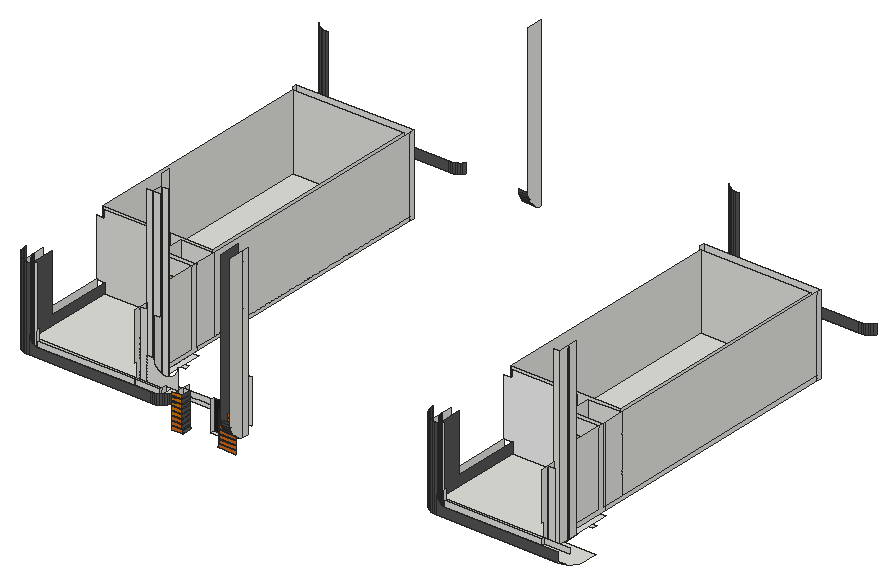
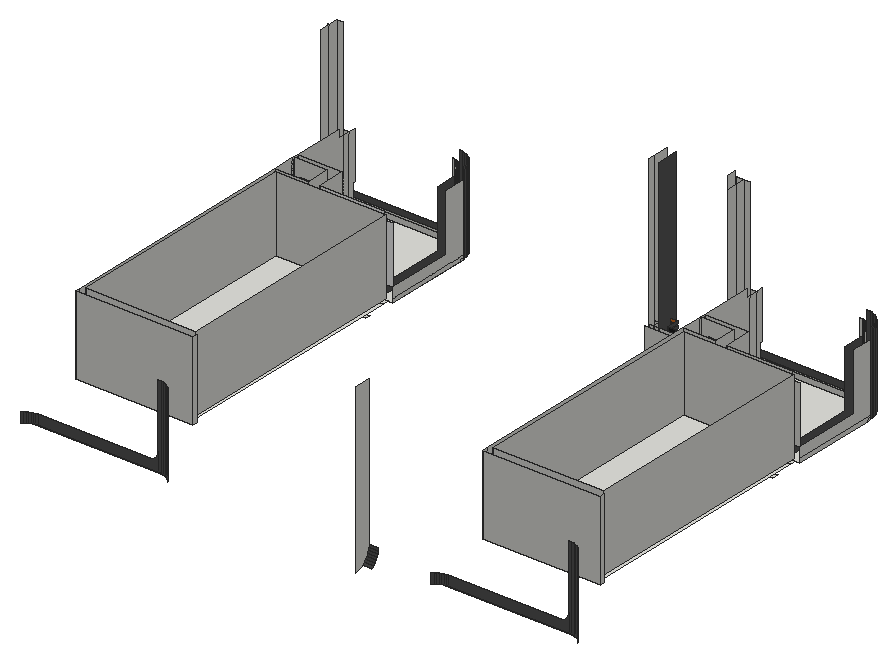
# SketchUp Ruby script. Lengths in inches.
U = 1.inch
M = Sketchup.active_model
def pt(a) = Geom::Point3d.new(a.map { |v| v * U })
def face(e, loops, mat)
  f = e.add_face(loops[0].map { |a| pt(a) })
  loops[1..].each { |l| e.add_face(l.map { |a| pt(a) }).erase! }
  f.material = f.back_material = mat if mat
  f
end
# faces: each face lists its corners as indices into pts; further lists are holes
def faces(e, pts, list, mat = nil) = list.each { |f| face(e, (f[0].is_a?(Array) ? f : [f]).map { |l| l.map { |i| pts[i] } }, mat) }
# xy, xz, yz: faces in a plane at the given z, y or x. An outline is a flat list of corners, or four numbers for a rectangle; further outlines are holes
def ring(l) = l.size == 4 ? [[l[0], l[1]], [l[2], l[1]], [l[2], l[3]], [l[0], l[3]]] : l.each_slice(2).to_a
def flat(e, list, mat, &to3) = list.each { |f| face(e, (f[0].is_a?(Array) ? f : [f]).map { |l| ring(l).map { |u, v| to3.(u, v) } }, mat) }
def xy(e, z, list, mat = nil) = flat(e, list, mat) { |x, y| [x, y, z] }
def xz(e, y, list, mat = nil) = flat(e, list, mat) { |x, z| [x, y, z] }
def yz(e, x, list, mat = nil) = flat(e, list, mat) { |y, z| [x, y, z] }
def lines(e, pts, list) = list.each { |a, b| e.add_line(pt(pts[a]), pt(pts[b])) }
# prism: a flat outline (further loops are holes) pulled along v
def prism(e, loops, v, mat = nil)
  f = face(e, loops, mat); d = Geom::Vector3d.new(v.map { |x| x * U })
  f.pushpull(f.normal.samedirection?(d) ? d.length : -d.length)
end
def box(e, o, s, mat = nil) = prism(e, [[o, [o[0] + s[0], o[1], o[2]], [o[0] + s[0], o[1] + s[1], o[2]], [o[0], o[1] + s[1], o[2]]]], [0, 0, s[2]], mat)
def at(x, y, z, deg = 0) = Geom::Transformation.translation(pt([x, y, z])) * Geom::Transformation.rotation(ORIGIN, Z_AXIS, deg.degrees)
def axes(o, x, y, z) = Geom::Transformation.new([*x, 0, *y, 0, *z, 0, *pt(o).to_a, 1])
def part(name) = M.definitions.add(name)
# library, detail: a bought-in or finely detailed component or shape, given as its bounding box
def library(name, o, s) = part(name).tap { |d| box(d.entities, o, s) }
def detail(e, o, s) = box(e.add_group.entities, o, s)
def put(e, d, t, mat = nil) = e.add_instance(d, t).tap { |i| i.material = mat if mat }
def group(e, t, mat = nil) = e.add_group.tap { |g| g.transformation = t; g.material = mat if mat }.entities
root = M.entities
M.materials.add("[0039_DarkOrange]").color = [219, 120, 0]
M.materials.add("[0041_Chocolate]").color = [210, 105, 30]
M.materials.add("[0129_WhiteSmoke]").color = [245, 245, 245]
M.materials.add("[Color M06]").color = [84, 84, 84]
M.materials.add("[Color M08]").color = [30, 30, 30]
c1 = library("元件\#5",[-4.39,0,0],[5.37,35.83,90.55])
xy(root,90.875,[[897.21,280.47,915.39,281.47],[969.37,280.47,998.64,281.47]],"[0041_Chocolate]")
xy(root,95.51,[[684.87,439.98,732.5,448.51],[1335.37,439.98,1383,448.51]])
xy(root,95.83,[[897.21,280.47,913.53,281.47],[971.24,280.47,998.64,281.47]],"[0041_Chocolate]")
xy(root,97.27,[[946.98,295.65,971.43,300.34]])
xy(root,97.9375,[[897.21,280.47,913.25,281.47],[971.52,280.47,998.64,281.47]],"[0041_Chocolate]")
xy(root,101.1875,[[777.42,397.86,824.61,405.05],[1427.92,397.86,1475.11,405.05]])
xy(root,102.89,[[897.21,280.47,912.6,281.47],[972.17,280.47,998.64,281.47]],"[0041_Chocolate]")
xy(root,105,[[897.21,280.47,912.6,281.47],[972.17,280.47,998.64,281.47]],"[0041_Chocolate]")
xy(root,109.9375,[[984.18,299.11,999.52,302.46]])
xy(root,109.95,[[897.21,280.47,912.6,281.47],[972.17,280.47,998.64,281.47]],"[0041_Chocolate]")
xy(root,112.0625,[[897.21,280.47,912.6,281.47]],"[0039_DarkOrange]")
xy(root,112.0625,[[972.17,280.47,998.64,281.47]],"[0041_Chocolate]")
xy(root,117.02,[[897.21,280.47,912.6,281.47]],"[0039_DarkOrange]")
xy(root,117.02,[[972.17,280.47,998.64,281.47]],"[0041_Chocolate]")
xy(root,119.125,[[897.21,280.47,912.6,281.47]],"[0039_DarkOrange]")
xy(root,119.125,[[972.17,280.47,998.64,281.47]],"[0041_Chocolate]")
xy(root,124.08,[[897.21,280.47,912.6,281.47]],"[0039_DarkOrange]")
xy(root,124.08,[[972.17,280.47,998.64,281.47]],"[0041_Chocolate]")
xy(root,126.125,[[679.54,267.75,675.54,268.01,671.61,268.79,669.16,269.625,881.95,269.625,878.9,268.59,875.73,267.96,872.51,267.75],[1330.04,267.75,1326.04,268.01,1322.11,268.79,1319.66,269.625,1532.45,269.625,1529.4,268.59,1526.23,267.96,1523.01,267.75],[669.16,269.625,667.8125,270.08,664.22,271.85,660.88,274.08,657.87,276.72,656.13,278.71,655.23,279.74,653,283.07,651.23,286.66,649.94,290.46,649.16,294.39,648.9,298.39,648.9,439.98,767.38,439.98,767.38,397.86,836,397.86,836,305.58,845.71,305.58,845.71,312.8125,897.21,312.8125,897.21,305.58,896.71,305.58,896.71,292.45,897.21,292.45,897,289.23,896.37,286.06,895.33,283,893.9,280.1,892.11,277.41,889.98,274.98,887.55,272.85,884.86,271.06,881.96,269.63,881.95,269.625],[1319.66,269.625,1318.3125,270.08,1314.72,271.85,1311.38,274.08,1308.37,276.72,1306.63,278.71,1305.73,279.74,1303.5,283.07,1301.73,286.66,1300.44,290.46,1299.66,294.39,1299.4,298.39,1299.4,439.98,1417.88,439.98,1417.88,397.86,1486.5,397.86,1486.5,305.58,1496.21,305.58,1496.21,312.8125,1547.71,312.8125,1547.71,305.58,1547.21,305.58,1547.21,292.45,1547.71,292.45,1547.5,289.23,1546.87,286.06,1545.83,283,1544.4,280.1,1542.61,277.41,1540.48,274.98,1538.05,272.85,1535.36,271.06,1532.46,269.63,1532.45,269.625],[896.71,292.45,897.21,302.46],
  [896.71,302.46,897.21,305.58],[836,305.58,845.71,312.8125],[1486.5,305.58,1496.21,312.8125],[836,312.8125,845.71,397.86],[845.71,312.8125,846.02,321.34],
  [846.02,312.8125,847.59,321.34],[847.59,312.8125,857.24,321.34],[857.24,312.8125,897.21,321.34],[1486.5,312.8125,1496.21,397.86],[1496.21,312.8125,1496.52,321.34],
  [1496.52,312.8125,1498.09,321.34],[845.71,321.34,846.02,336.27],[846.02,321.34,847.59,336.27],[1496.21,321.34,1496.52,336.27],[1496.52,321.34,1498.09,336.27],
  [767.38,397.86,786.21,397.86,786.21,448.51,656.13,448.51,656.13,439.98,767.38,439.98],[786.21,397.86,836,406.38],[1417.88,397.86,1436.71,397.86,1436.71,448.51,1306.63,448.51,1306.63,439.98,1417.88,439.98],[1436.71,397.86,1486.5,406.38],[786.21,406.38,836,830.91],
  [1436.71,406.38,1486.5,830.91],[656.13,448.51,786.21,830.91],[1306.63,448.51,1436.71,830.91],[648.9,830.91,836,838.14],[1299.4,830.91,1486.5,838.14],
  [602.85,958.64,598.85,958.91,594.92,959.6875,592.47,960.52,805.26,960.52,802.22,959.49,799.05,958.86,795.82,958.64],[1258.35,958.64,1254.35,958.91,1250.42,959.6875,1247.97,960.52,1460.76,960.52,1457.72,959.49,1454.55,958.86,1451.32,958.64]])
xy(root,126.1875,[[897.21,280.47,912.6,281.47]],"[0039_DarkOrange]")
xy(root,126.1875,[[972.17,280.47,998.64,281.47]],"[0041_Chocolate]")
xy(root,128.75,[[648.9,294.33,661.9,305.58],[1299.4,294.33,1312.4,305.58]])
xy(root,131.14,[[897.21,280.47,912.6,281.47]],"[0039_DarkOrange]")
xy(root,131.14,[[972.17,280.47,998.64,281.47]],"[0041_Chocolate]")
xy(root,132.47,[[679.54,281.47,679.54,285.84,836,285.84,836,395.98,824.61,395.98,824.61,403.17,777.42,403.17,777.42,395.98,765.68,395.98,765.68,439.98,662.61,439.98,662.61,298.39,662.76,296.18,663.1875,294.01,663.9,291.91,664.88,289.93,666.11,288.09,667.57,286.42,669.23,284.96,671.07,283.73,673.06,282.75,675.16,282.04,677.33,281.61],[679.54,281.47,836,285.84],[836,281.47,876.59,285.84],[1330.04,281.47,1330.04,285.84,1486.5,285.84,1486.5,395.98,1475.11,395.98,1475.11,403.17,1427.92,403.17,1427.92,395.98,1416.18,395.98,1416.18,439.98,1313.11,439.98,1313.11,298.39,1313.26,296.18,1313.6875,294.01,1314.4,291.91,1315.38,289.93,1316.61,288.09,1318.07,286.42,1319.73,284.96,1321.57,283.73,1323.56,282.75,1325.66,282.04,1327.83,281.61],[1330.04,281.47,1486.5,285.84],
  [836,285.84,876.59,292.45],[836,292.45,876.59,312.8125],[783.26,403.17,836,439.98],[1433.76,403.17,1486.5,439.98],[654.4,445.49,830.5,825.41],
  [1304.9,445.49,1481,825.41]])
xy(root,133.25,[[897.21,280.47,912.6,281.47]],"[0039_DarkOrange]")
xy(root,133.25,[[972.17,280.47,998.64,281.47]],"[0041_Chocolate]")
xy(root,138.2,[[897.21,280.47,912.6,281.47]],"[0039_DarkOrange]")
xy(root,138.2,[[972.17,280.47,998.64,281.47]],"[0041_Chocolate]")
xy(root,140.3125,[[897.21,280.47,912.6,281.47]],"[0039_DarkOrange]")
xy(root,140.3125,[[972.17,280.47,998.64,281.47]],"[0041_Chocolate]")
xz(root,267.75,[[679.54,126.125,872.51,126.125,872.51,141.26,692.98,141.26,691.2,141.46,689.46,141.89,687.79,142.53,686.21,143.38,684.75,144.42,683.43,145.64,682.28,147.01,681.32,148.52,680.55,150.14,679.99,151.84,679.65,153.6,679.54,155.39],[1330.04,126.125,1523.01,126.125,1523.01,141.26,1343.48,141.26,1341.7,141.46,1339.96,141.89,1338.29,142.53,1336.71,143.38,1335.25,144.42,1333.93,145.64,1332.78,147.01,1331.82,148.52,1331.05,150.14,1330.49,151.84,1330.15,153.6,1330.04,155.39]],"[Color M06]")
xz(root,280.47,[[897.21,112.0625,912.6,117.02],[897.21,119.125,912.6,124.08],[897.21,126.1875,912.6,131.14],[897.21,133.25,912.6,138.2],[897.21,140.3125,912.6,145.27]],"[0039_DarkOrange]")
xz(root,280.47,[[897.21,90.875,915.39,90.875,913.61,95.18,913.53,95.83,897.21,95.83],[969.37,90.875,998.64,90.875,998.64,95.83,971.24,95.83,971.16,95.18],[897.21,97.9375,913.25,97.9375,912.6,102.89,897.21,102.89],[971.52,97.9375,998.64,97.9375,998.64,102.89,972.17,102.89],[897.21,105,912.6,109.95],
  [972.17,105,998.64,109.95],[972.17,112.0625,998.64,117.02],[972.17,119.125,998.64,124.08],[972.17,126.1875,998.64,131.14],[972.17,133.25,998.64,138.2],
  [972.17,140.3125,998.64,145.27]],"[0041_Chocolate]")
xz(root,281.47,[[679.54,132.47,836,141.26],[836,132.47,876.59,141.26],[1330.04,132.47,1486.5,141.26]])
xz(root,281.47,[[897.21,117.02,912.6,119.125],[897.21,124.08,912.6,126.1875],[897.21,131.14,912.6,133.25],[897.21,138.2,912.6,140.3125]],"[0039_DarkOrange]")
xz(root,281.47,[[897.21,95.83,913.53,95.83,913.25,97.9375,897.21,97.9375],[971.24,95.83,998.64,95.83,998.64,97.9375,971.52,97.9375],[897.21,102.89,912.6,105],[972.17,102.89,998.64,105],[897.21,109.95,912.6,112.0625],
  [972.17,109.95,998.64,112.0625],[972.17,117.02,998.64,119.125],[972.17,124.08,998.64,126.1875],[972.17,131.14,998.64,133.25],[972.17,138.2,998.64,140.3125]],"[0041_Chocolate]")
xz(root,285.84,[[679.54,132.47,876.59,141.26],[1330.04,132.47,1527.09,141.26]])
xz(root,292.45,[[991.85,126.125,992.73,141.26],[992.73,126.125,998.64,141.26],[836,132.47,847.59,240.16],[847.59,132.47,876.59,132.47,876.59,141.26,897.21,141.26,897.21,174.51,897.18,173.46,897.1,172.42,896.96,171.38,896.77,170.36,896.53,169.34,896.23,168.33,895.88,167.35,895.48,166.38,895.03,165.4375,894.53,164.52,893.99,163.625,893.39,162.76,892.76,161.93,892.08,161.14,891.36,160.38,890.6,159.66,889.8,158.98,888.97,158.34,888.11,157.75,887.22,157.2,886.3,156.7,885.36,156.25,884.39,155.85,883.4,155.5,882.4,155.21,881.38,154.96,880.35,154.77,879.32,154.64,878.27,154.55,877.23,154.53,876.18,154.55,875.14,154.64,874.1,154.77,873.07,154.96,872.05,155.21,871.05,155.5,870.07,155.85,869.1,156.25,868.15,156.7,867.23,157.2,866.34,157.75,865.48,158.34,864.65,158.98,863.85,159.66,863.1,160.38,862.375,161.14,861.7,161.93,861.06,162.76,860.47,163.625,859.92,164.52,859.42,165.4375,858.97,166.38,858.57,167.35,858.22,168.33,857.92,169.34,857.68,170.36,857.49,171.38,857.35,172.42,857.27,173.46,857.24,174.51,847.59,174.51],[1486.5,132.47,1498.09,240.16]])
xz(root,295.65,[[971.43,97.27,972.17,97.27,972.17,102.89,971.52,97.9375]])
xz(root,300.34,[[946.98,97.27,971.43,97.27,971.52,97.9375,972.17,102.89,972.17,145.27,946.98,145.27]],"[Color M08]")
xz(root,302.46,[[896.71,95.62,897.21,126.125],[984.18,109.9375,991.85,126.125],[991.85,109.9375,992.73,126.125],[992.73,109.9375,999.52,126.125],[897.21,126.125,984.18,132.47],
  [984.18,126.125,991.85,132.47],[991.85,126.125,992.73,132.47],[992.73,126.125,999.52,132.47],[897.21,132.47,984.18,141.26],[984.18,132.47,991.85,141.26],
  [991.85,132.47,992.73,141.26],[992.73,132.47,999.52,141.26]])
xz(root,305.58,[[836,126.125,845.71,402.64],[845.71,126.125,847.59,126.125,847.59,226.8,857.24,226.8,857.24,402.64,845.71,402.64],[1486.5,126.125,1496.21,402.64]])
xz(root,312.8125,[[836,126.125,897.21,132.47]])
xz(root,321.34,[[845.71,126.125,847.59,402.64],[847.59,126.125,857.24,402.64],[1496.21,126.125,1498.09,402.64]])
xz(root,343.15,[[937.76,96.14,974.45,165.14]])
xz(root,395.98,[[765.68,132.47,777.42,132.47,777.42,227.53,824.61,227.53,824.61,132.47,836,132.47,836,252.47,765.68,252.47],[1416.18,132.47,1427.92,132.47,1427.92,227.53,1475.11,227.53,1475.11,132.47,1486.5,132.47,1486.5,252.47,1416.18,252.47]])
xz(root,403.17,[[777.42,132.47,783.26,227.53],[783.26,132.47,824.61,227.53],[824.61,132.47,824.61,227.53,783.26,227.53,783.26,252.47,836,252.47,836,132.47],[1427.92,132.47,1433.76,227.53],[1433.76,132.47,1475.11,227.53],
  [1475.11,132.47,1475.11,227.53,1433.76,227.53,1433.76,252.47,1486.5,252.47,1486.5,132.47]])
xz(root,439.98,[[662.61,132.47,765.68,132.47,765.68,252.47,662.61,252.47,662.61,240.16,648.9,240.16,648.9,148.66,662.61,148.66],[783.26,132.47,836,252.47],[1433.76,132.47,1486.5,252.47]])
xz(root,439.98,[[1313.11,132.47,1416.18,132.47,1416.18,252.47,1313.11,252.47,1313.11,240.16,1299.4,240.16,1299.4,148.66,1313.11,148.66]],"[0129_WhiteSmoke]")
xz(root,445.49,[[654.4,132.47,830.5,252.47],[1304.9,132.47,1481,252.47]])
xz(root,825.41,[[654.4,132.47,830.5,252.47],[1304.9,132.47,1481,252.47]])
xz(root,838.14,[[648.9,126.125,836,252.47],[1299.4,126.125,1486.5,252.47]])
xz(root,958.64,[[602.85,126.125,795.82,126.125,795.82,141.26,616.29,141.26,614.51,141.46,612.77,141.89,611.1,142.53,609.52,143.38,608.0625,144.42,606.75,145.64,605.6,147.01,604.63,148.52,603.86,150.14,603.3,151.84,602.96,153.6,602.85,155.39],[1258.35,126.125,1451.32,126.125,1451.32,141.26,1271.79,141.26,1270.01,141.46,1268.27,141.89,1266.6,142.53,1265.02,143.38,1263.5625,144.42,1262.25,145.64,1261.1,147.01,1260.13,148.52,1259.36,150.14,1258.8,151.84,1258.46,153.6,1258.35,155.39]],"[Color M06]")
yz(root,648.9,[[298.39,126.125,305.58,128.75],[305.58,126.125,305.58,128.75,298.39,128.75,298.39,132.47,439.98,132.47,439.98,126.125],[830.91,126.125,838.14,252.47],[298.39,132.47,298.39,240.16,333.33,240.16,333.33,148.66,439.98,148.66,439.98,132.47]])
yz(root,654.4,[[445.49,132.47,825.41,252.47]])
yz(root,662.61,[[298.39,132.47,439.98,132.47,439.98,148.66,333.33,148.66,333.33,240.16,298.39,240.16]],"[Color M06]")
yz(root,679.54,[[281.47,132.47,285.84,155.39]])
yz(root,765.68,[[395.98,132.47,439.98,252.47]])
yz(root,777.42,[[395.98,132.47,403.17,227.53]])
yz(root,783.26,[[403.17,132.47,439.98,252.47]])
yz(root,824.61,[[395.98,132.47,403.17,227.53]])
yz(root,830.5,[[445.49,132.47,825.41,252.47]])
yz(root,836,[[312.8125,126.125,312.8125,132.47,395.98,132.47,395.98,252.47,403.17,252.47,403.17,132.47,406.38,132.47,406.38,126.125],[406.38,126.125,830.91,132.47],[830.91,126.125,838.14,252.47],[281.47,132.47,281.47,141.26,285.84,141.26,285.84,163.7,281.47,163.7,281.47,240.16,292.45,240.16,292.45,132.47],[292.45,132.47,305.58,240.16],
  [305.58,132.47,305.58,240.16,312.8125,240.16,312.8125,252.47,395.98,252.47,395.98,132.47],[403.17,132.47,406.38,252.47],[406.38,132.47,439.98,252.47],[439.98,132.47,830.91,252.47]])
yz(root,845.71,[[305.58,126.125,321.34,402.64],[321.34,126.125,337.5625,402.64]])
yz(root,847.59,[[321.34,126.125,336.27,421.25]])
yz(root,876.59,[[281.47,132.47,285.84,141.26],[285.84,132.47,292.45,141.26]])
yz(root,896.71,[[302.46,95.62,305.58,126.125]])
yz(root,897.21,[[292.45,126.125,302.46,141.26],[302.46,126.125,305.58,132.47],[305.58,126.125,312.8125,132.47],[302.46,132.47,305.58,141.26],[305.58,132.47,312.8125,141.26]])
yz(root,912.6,[[281.47,102.89,295.65,105],[280.47,105,295.65,109.95],[281.47,109.95,295.65,112.0625],[280.47,112.0625,295.65,117.02],[281.47,117.02,295.65,119.125],
  [280.47,119.125,295.65,124.08],[281.47,124.08,295.65,126.1875],[280.47,126.1875,295.65,131.14],[281.47,131.14,295.65,133.25],[280.47,133.25,295.65,138.2],
  [281.47,138.2,295.65,140.3125],[280.47,140.3125,295.65,145.27]],"[Color M06]")
yz(root,922.83,[[983.34,110.72,983.34,376.875,958.64,376.875,958.64,141.3,958.91,137.2,959.71,133.18,961.03,129.3,962.85,125.62,965.125,122.21,967.83,119.12,970.91,116.42,974.32,114.14,978,112.32,981.89,111.01]])
yz(root,946.98,[[295.65,97.27,300.34,145.27]])
yz(root,972.17,[[281.47,102.89,300.34,105],[280.47,105,300.34,109.95],[281.47,109.95,300.34,112.0625],[280.47,112.0625,300.34,117.02],[281.47,117.02,300.34,119.125],
  [280.47,119.125,300.34,124.08],[281.47,124.08,300.34,126.1875],[280.47,126.1875,300.34,131.14],[281.47,131.14,300.34,133.25],[280.47,133.25,300.34,138.2],
  [281.47,138.2,300.34,140.3125],[280.47,140.3125,300.34,145.27]],"[Color M06]")
yz(root,984.18,[[299.11,109.9375,295.02,110.21,290.99,111.01,287.11,112.32,283.43,114.14,280.02,116.42,276.93,119.12,274.23,122.21,271.95,125.62,270.14,129.3,268.82,133.18,268.02,137.2,267.75,141.3,267.75,376.875,302.46,376.875,302.46,109.9375]],"[Color M06]")
yz(root,991.85,[[292.45,126.125,302.46,141.26]])
yz(root,999.52,[[299.11,109.9375,302.46,109.9375,302.46,376.875,292.45,376.875,292.45,110.72,295.02,110.21],[292.45,110.72,292.45,376.875,267.75,376.875,267.75,141.3,268.02,137.2,268.82,133.18,270.14,129.3,271.95,125.62,274.23,122.21,276.93,119.12,280.02,116.42,283.43,114.14,287.11,112.32,290.99,111.01]])
yz(root,1299.4,[[298.39,126.125,305.58,128.75],[305.58,126.125,305.58,128.75,298.39,128.75,298.39,132.47,439.98,132.47,439.98,126.125],[830.91,126.125,838.14,252.47],[298.39,132.47,298.39,240.16,333.33,240.16,333.33,148.66,439.98,148.66,439.98,132.47]])
yz(root,1304.9,[[445.49,132.47,825.41,252.47]])
yz(root,1313.11,[[298.39,132.47,439.98,132.47,439.98,148.66,333.33,148.66,333.33,240.16,298.39,240.16]],"[Color M06]")
yz(root,1330.04,[[281.47,132.47,285.84,155.39]])
yz(root,1416.18,[[395.98,132.47,439.98,252.47]])
yz(root,1427.92,[[395.98,132.47,403.17,227.53]])
yz(root,1433.76,[[403.17,132.47,439.98,252.47]])
yz(root,1475.11,[[395.98,132.47,403.17,227.53]])
yz(root,1481,[[445.49,132.47,825.41,252.47]])
yz(root,1486.5,[[312.8125,126.125,312.8125,132.47,395.98,132.47,395.98,252.47,403.17,252.47,403.17,132.47,406.38,132.47,406.38,126.125],[406.38,126.125,830.91,132.47],[830.91,126.125,838.14,252.47],[281.47,132.47,281.47,141.26,285.84,141.26,285.84,163.7,281.47,163.7,281.47,240.16,292.45,240.16,292.45,132.47],[292.45,132.47,305.58,240.16],
  [305.58,132.47,305.58,240.16,312.8125,240.16,312.8125,252.47,395.98,252.47,395.98,132.47],[403.17,132.47,406.38,252.47],[406.38,132.47,439.98,252.47],[439.98,132.47,830.91,252.47]])
yz(root,1496.21,[[305.58,126.125,321.34,402.64],[321.34,126.125,337.5625,402.64]])
p = [[913.61,295.65,95.18],[913.61,280.47,95.18],[915.39,280.47,90.875],[915.39,281.47,90.875],[915.39,295.65,90.875],[969.37,295.65,90.875],
  [969.37,281.47,90.875],[969.37,280.47,90.875],[971.16,280.47,95.18],[971.16,295.65,95.18],[913.53,295.65,95.83],[913.53,281.47,95.83],
  [913.53,280.47,95.83],[971.24,280.47,95.83],[971.24,281.47,95.83],[971.24,295.65,95.83],[913.25,281.47,97.9375],[913.25,295.65,97.9375],
  [971.52,281.47,97.9375],[971.52,295.65,97.9375],[971.43,295.65,97.27],[971.52,300.34,97.9375],[971.43,300.34,97.27],[912.6,295.65,102.89],
  [912.6,281.47,102.89],[912.6,280.47,102.89],[913.25,280.47,97.9375],[971.52,280.47,97.9375],[972.17,280.47,102.89],[972.17,281.47,102.89],
  [972.17,295.65,102.89],[972.17,300.34,102.89],[999.52,299.11,109.9375],[999.52,295.02,110.21],[984.18,295.02,110.21],[984.18,299.11,109.9375],
  [999.52,292.45,110.72],[999.52,290.99,111.01],[984.18,290.99,111.01],[999.52,287.11,112.32],[984.18,287.11,112.32],[999.52,283.43,114.14],
  [984.18,283.43,114.14],[999.52,280.02,116.42],[984.18,280.02,116.42],[999.52,276.93,119.12],[984.18,276.93,119.12],[922.83,970.91,116.42],
  [922.83,967.83,119.12],[907.49,967.83,119.12],[907.49,970.91,116.42],[999.52,274.23,122.21],[984.18,274.23,122.21],[922.83,965.125,122.21],
  [907.49,965.125,122.21],[999.52,271.95,125.62],[984.18,271.95,125.62],[922.83,962.85,125.62],[907.49,962.85,125.62],[999.52,270.14,129.3],
  [984.18,270.14,129.3],[922.83,961.03,129.3],[907.49,961.03,129.3],[679.54,267.75,258.13],[675.54,268.01,258.13],[675.54,268.01,126.125],
  [679.54,267.75,126.125],[679.54,267.75,155.39],[679.54,267.75,164.97],[679.54,267.75,240.16],[875.73,267.96,141.26],[872.51,267.75,141.26],
  [872.51,267.75,126.125],[875.73,267.96,126.125],[1330.04,267.75,258.13],[1326.04,268.01,258.13],[1326.04,268.01,126.125],[1330.04,267.75,126.125],
  [1330.04,267.75,155.39],[1330.04,267.75,164.97],[1330.04,267.75,240.16],[671.61,268.79,258.13],[671.61,268.79,126.125],[878.9,268.59,141.26],
  [878.9,268.59,126.125],[1322.11,268.79,258.13],[1322.11,268.79,126.125],[881.96,269.63,141.26],[881.95,269.625,126.125],[881.96,269.63,126.125],
  [667.8125,270.08,258.13],[667.8125,270.08,126.125],[669.16,269.625,126.125],[1318.3125,270.08,258.13],[1318.3125,270.08,126.125],[1319.66,269.625,126.125],
  [884.86,271.06,141.26],[884.86,271.06,126.125],[664.22,271.85,258.13],[664.22,271.85,126.125],[1314.72,271.85,258.13],[1314.72,271.85,126.125],
  [887.55,272.85,141.26],[887.55,272.85,126.125],[660.88,274.08,258.13],[660.88,274.08,126.125],[1311.38,274.08,258.13],[1311.38,274.08,126.125],
  [889.98,274.98,141.26],[889.98,274.98,126.125],[657.87,276.72,258.13],[657.87,276.72,126.125],[1308.37,276.72,258.13],[1308.37,276.72,126.125],
  [892.11,277.41,141.26],[892.11,277.41,126.125],[655.23,279.74,258.13],[655.23,279.74,126.125],[656.13,278.71,126.125],[1305.73,279.74,258.13],
  [1305.73,279.74,126.125],[1306.63,278.71,126.125],[893.9,280.1,141.26],[893.9,280.1,126.125],[653,283.07,258.13],[653,283.07,126.125],
  [1303.5,283.07,258.13],[1303.5,283.07,126.125],[894.57,281.47,141.26],[895.33,283,126.125],[895.33,283,141.26],[896.37,286.06,141.26],
  [896.37,286.06,126.125],[651.23,286.66,258.13],[651.23,286.66,126.125],[1301.73,286.66,258.13],[1301.73,286.66,126.125],[897,289.23,141.26],
  [897,289.23,126.125],[649.94,290.46,258.13],[649.94,290.46,126.125],[1300.44,290.46,258.13],[1300.44,290.46,126.125],[897.21,292.45,141.26],
  [897.21,292.45,126.125],[649.16,294.39,258.13],[649.16,294.39,126.125],[1299.66,294.39,258.13],[1299.66,294.39,126.125],[648.9,298.39,240.16],
  [648.9,298.39,132.47],[648.9,298.39,128.75],[648.9,298.39,126.125],[648.9,298.39,258.13],[1299.4,298.39,240.16],[1299.4,298.39,132.47],
  [1299.4,298.39,128.75],[1299.4,298.39,126.125],[1299.4,298.39,258.13],[602.85,958.64,258.13],[598.85,958.91,258.13],[598.85,958.91,126.125],
  [602.85,958.64,126.125],[602.85,958.64,155.39],[602.85,958.64,164.97],[602.85,958.64,240.16],[799.05,958.86,141.26],[795.82,958.64,141.26],
  [795.82,958.64,126.125],[799.05,958.86,126.125],[1258.35,958.64,258.13],[1254.35,958.91,258.13],[1254.35,958.91,126.125],[1258.35,958.64,126.125],
  [1258.35,958.64,155.39],[1258.35,958.64,164.97],[1258.35,958.64,240.16],[1454.55,958.86,141.26],[1451.32,958.64,141.26],[1451.32,958.64,126.125],
  [1454.55,958.86,126.125],[594.92,959.6875,258.13],[594.92,959.6875,126.125],[802.22,959.49,141.26],[802.22,959.49,126.125],[1250.42,959.6875,258.13],
  [1250.42,959.6875,126.125],[1457.72,959.49,141.26],[1457.72,959.49,126.125],[805.28,960.52,141.26],[805.26,960.52,126.125],[805.28,960.52,126.125],
  [1460.78,960.52,141.26],[1460.76,960.52,126.125],[1460.78,960.52,126.125],[591.125,960.98,258.13],[591.125,960.98,126.125],[592.47,960.52,126.125],
  [1246.625,960.98,258.13],[1246.625,960.98,126.125],[1247.97,960.52,126.125],[808.17,961.95,141.26],[808.17,961.95,126.125],[1463.67,961.95,141.26],
  [1463.67,961.95,126.125],[587.53,962.75,258.13],[587.53,962.75,126.125],[1243.03,962.75,258.13],[1243.03,962.75,126.125],[810.86,963.75,141.26],
  [810.86,963.75,126.125],[1466.36,963.75,141.26],[1466.36,963.75,126.125],[584.2,964.98,258.13],[584.2,964.98,126.125],[1239.7,964.98,258.13],
  [1239.7,964.98,126.125],[813.29,965.88,141.26],[813.29,965.88,126.125],[1468.79,965.88,141.26],[1468.79,965.88,126.125],[581.18,967.62,258.13],
  [581.18,967.62,126.125],[1236.68,967.62,258.13],[1236.68,967.62,126.125],[815.42,968.31,141.26],[815.42,968.31,126.125],[1470.92,968.31,141.26],
  [1470.92,968.31,126.125],[578.54,970.63,258.13],[578.54,970.63,126.125],[579.44,969.61,126.125],[1234.04,970.63,258.13],[1234.04,970.63,126.125],
  [1234.94,969.61,126.125],[999.52,268.82,133.18],[984.18,268.82,133.18],[922.83,959.71,133.18],[907.49,959.71,133.18],[677.33,281.61,252.47],
  [679.54,281.47,252.47],[679.54,281.47,240.16],[679.54,281.47,164.97],[679.54,281.47,163.7],[679.54,281.47,155.39],[679.54,281.47,141.26],
  [679.54,281.47,132.47],[677.33,281.61,132.47],[1327.83,281.61,252.47],[1330.04,281.47,252.47],[1330.04,281.47,240.16],[1330.04,281.47,164.97],
  [1330.04,281.47,163.7],[1330.04,281.47,155.39],[1330.04,281.47,141.26],[1330.04,281.47,132.47],[1327.83,281.61,132.47],[675.16,282.04,252.47],
  [675.16,282.04,132.47],[1325.66,282.04,252.47],[1325.66,282.04,132.47],[673.06,282.75,252.47],[673.06,282.75,132.47],[1323.56,282.75,252.47],
  [1323.56,282.75,132.47],[671.07,283.73,252.47],[671.07,283.73,132.47],[1321.57,283.73,252.47],[1321.57,283.73,132.47],[669.23,284.96,252.47],
  [669.23,284.96,132.47],[1319.73,284.96,252.47],[1319.73,284.96,132.47],[667.57,286.42,252.47],[667.57,286.42,132.47],[1318.07,286.42,252.47],
  [1318.07,286.42,132.47],[666.11,288.09,252.47],[666.11,288.09,132.47],[1316.61,288.09,252.47],[1316.61,288.09,132.47],[664.88,289.93,252.47],
  [664.88,289.93,132.47],[1315.38,289.93,252.47],[1315.38,289.93,132.47],[663.9,291.91,252.47],[663.9,291.91,132.47],[1314.4,291.91,252.47],
  [1314.4,291.91,132.47],[663.1875,294.01,252.47],[663.1875,294.01,132.47],[1313.6875,294.01,252.47],[1313.6875,294.01,132.47],[662.76,296.18,252.47],
  [662.76,296.18,132.47],[1313.26,296.18,252.47],[1313.26,296.18,132.47],[662.61,298.39,252.47],[662.61,298.39,132.47],[662.61,298.39,240.16],
  [1313.11,298.39,252.47],[1313.11,298.39,132.47],[1313.11,298.39,240.16],[999.52,268.02,137.2],[984.18,268.02,137.2],[922.83,958.91,137.2],
  [907.49,958.91,137.2],[999.52,267.75,141.3],[984.18,267.75,141.3],[922.83,958.64,141.3],[907.49,958.64,141.3],[974.45,321.34,96.14],
  [974.45,343.15,96.14],[937.76,321.34,96.14],[937.76,343.15,96.14]]
faces(root,p,[[0,1,2,3,4],[5,6,7,8,9],[10,11,12,1,0],[9,8,13,14,15],[16,11,10,17],[14,18,19,20,15],[23,24,25,26,16,17],[19,18,27,28,29,30],
  [19,30,31,21],[32,33,34,35],[36,37,38,34,33],[37,39,40,38],[39,41,42,40],[41,43,44,42],[43,45,46,44],[47,48,49,50],
  [45,51,52,46],[48,53,54,49],[51,55,56,52],[53,57,58,54],[55,59,60,56],[57,61,62,58],[63,64,65,66,67,68,69],[70,71,72,73],
  [74,75,76,77,78,79,80],[64,81,82,65],[83,70,73,84],[75,85,86,76],[87,83,84,88,89],[90,91,92,82,81],[93,94,95,86,85],[96,87,89,97],
  [98,99,91,90],[100,101,94,93],[102,96,97,103],[104,105,99,98],[106,107,101,100],[108,102,103,109],[110,111,105,104],[112,113,107,106],
  [114,108,109,115],[116,117,118,111,110],[119,120,121,113,112],[122,114,115,123],[124,125,117,116],[126,127,120,119],[128,122,123,129,130],[131,130,129,132],
  [133,134,125,124],[135,136,127,126],[137,131,132,138],[139,140,134,133],[141,142,136,135],[143,137,138,144],[145,146,140,139],[147,148,142,141],
  [149,150,151,152,146,145,153],[154,155,156,157,148,147,158],[159,160,161,162,163,164,165],[166,167,168,169],[170,171,172,173,174,175,176],[177,178,179,180],[160,181,182,161],[183,166,169,184],
  [171,185,186,172],[187,177,180,188],[189,183,184,190,191],[192,187,188,193,194],[195,196,197,182,181],[198,199,200,186,185],[201,189,191,202],[203,192,194,204],
  [205,206,196,195],[207,208,199,198],[209,201,202,210],[211,203,204,212],[213,214,206,205],[215,216,208,207],[217,209,210,218],[219,211,212,220],
  [221,222,214,213],[223,224,216,215],[225,217,218,226],[227,219,220,228],[229,230,231,222,221],[232,233,234,224,223],[59,235,236,60],[61,237,238,62],
  [235,303,304,236],[237,305,306,238],[303,307,308,304],[305,309,310,306]],"[Color M06]")
faces(root,p,[[20,19,21,22],[239,240,241,242,243,244,245,246,247],[248,249,250,251,252,253,254,255,256],[257,239,247,258],[259,248,256,260],[261,257,258,262],[263,259,260,264],[265,261,262,266],
  [267,263,264,268],[269,265,266,270],[271,267,268,272],[273,269,270,274],[275,271,272,276],[277,273,274,278],[279,275,276,280],[281,277,278,282],
  [283,279,280,284],[285,281,282,286],[287,283,284,288],[289,285,286,290],[291,287,288,292],[293,289,290,294],[295,291,292,296],[297,293,294,298,299],
  [300,295,296,301,302]])
lines(root,p,[[311,312],[313,314]])
put(root,c1,axes([777.42,396.14,132.47],[0,-1.05,0],[1.302,0,0],[0,0,1.05]))
put(root,c1,axes([1427.92,396.14,132.47],[0,-1.05,0],[1.302,0,0],[0,0,1.05]))
